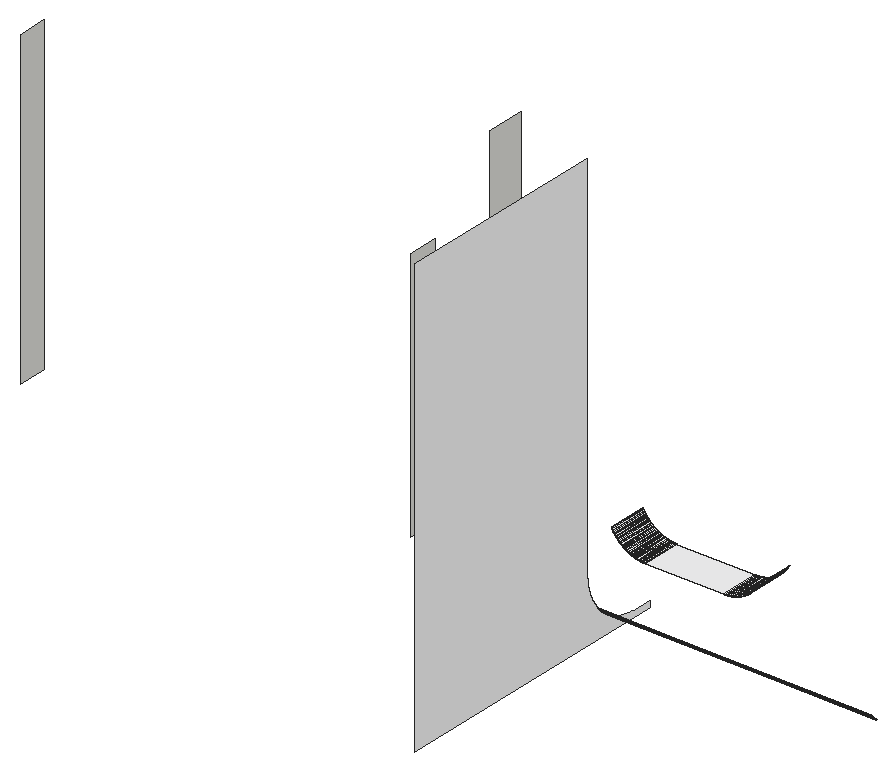
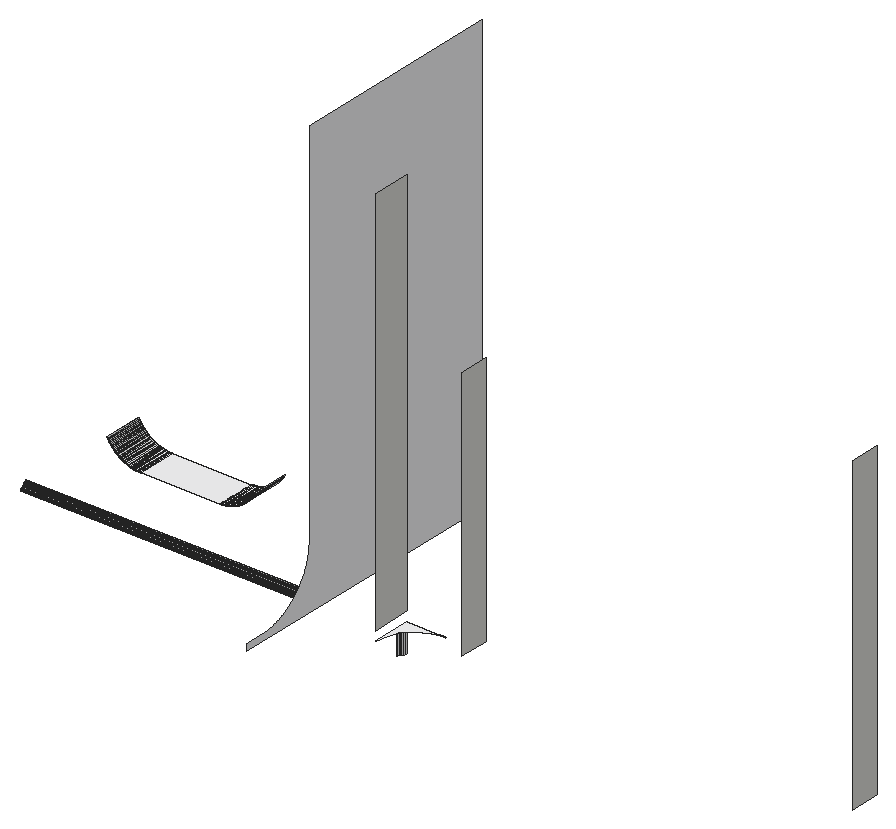
# SketchUp Ruby script. Lengths in inches.
U = 1.inch
M = Sketchup.active_model
def pt(a) = Geom::Point3d.new(a.map { |v| v * U })
def face(e, loops, mat)
  f = e.add_face(loops[0].map { |a| pt(a) })
  loops[1..].each { |l| e.add_face(l.map { |a| pt(a) }).erase! }
  f.material = f.back_material = mat if mat
  f
end
# faces: each face lists its corners as indices into pts; further lists are holes
def faces(e, pts, list, mat = nil) = list.each { |f| face(e, (f[0].is_a?(Array) ? f : [f]).map { |l| l.map { |i| pts[i] } }, mat) }
# xy, xz, yz: faces in a plane at the given z, y or x. An outline is a flat list of corners, or four numbers for a rectangle; further outlines are holes
def ring(l) = l.size == 4 ? [[l[0], l[1]], [l[2], l[1]], [l[2], l[3]], [l[0], l[3]]] : l.each_slice(2).to_a
def flat(e, list, mat, &to3) = list.each { |f| face(e, (f[0].is_a?(Array) ? f : [f]).map { |l| ring(l).map { |u, v| to3.(u, v) } }, mat) }
def xy(e, z, list, mat = nil) = flat(e, list, mat) { |x, y| [x, y, z] }
def xz(e, y, list, mat = nil) = flat(e, list, mat) { |x, z| [x, y, z] }
def yz(e, x, list, mat = nil) = flat(e, list, mat) { |y, z| [x, y, z] }
def lines(e, pts, list) = list.each { |a, b| e.add_line(pt(pts[a]), pt(pts[b])) }
# prism: a flat outline (further loops are holes) pulled along v
def prism(e, loops, v, mat = nil)
  f = face(e, loops, mat); d = Geom::Vector3d.new(v.map { |x| x * U })
  f.pushpull(f.normal.samedirection?(d) ? d.length : -d.length)
end
def box(e, o, s, mat = nil) = prism(e, [[o, [o[0] + s[0], o[1], o[2]], [o[0] + s[0], o[1] + s[1], o[2]], [o[0], o[1] + s[1], o[2]]]], [0, 0, s[2]], mat)
def at(x, y, z, deg = 0) = Geom::Transformation.translation(pt([x, y, z])) * Geom::Transformation.rotation(ORIGIN, Z_AXIS, deg.degrees)
def axes(o, x, y, z) = Geom::Transformation.new([*x, 0, *y, 0, *z, 0, *pt(o).to_a, 1])
def part(name) = M.definitions.add(name)
# library, detail: a bought-in or finely detailed component or shape, given as its bounding box
def library(name, o, s) = part(name).tap { |d| box(d.entities, o, s) }
def detail(e, o, s) = box(e.add_group.entities, o, s)
def put(e, d, t, mat = nil) = e.add_instance(d, t).tap { |i| i.material = mat if mat }
def group(e, t, mat = nil) = e.add_group.tap { |g| g.transformation = t; g.material = mat if mat }.entities
root = M.entities
M.materials.add("[Quartz Light Grey]").color = [251, 251, 252]
xy(root,123,[[186,271,198,271,198,283,198,282.6875,197.99,282.53,197.98,282.37,197.97,282.22,197.95,281.9,197.93,281.75,197.92,281.59,197.9,281.43,197.875,281.28,197.85,281.12,197.83,280.97,197.8,280.8125,197.77,280.66,197.74,280.51,197.7,280.35,197.67,280.2,197.63,280.05,197.59,279.89,197.51,279.59,197.36,279.14,197.3125,278.99,197.26,278.85,197.2,278.7,197.15,278.55,197.09,278.41,197.03,278.26,196.96,278.12,196.9,277.98,196.83,277.83,196.55,277.27,196.47,277.14,196.39,277,196.3125,276.86,196.23,276.73,196.15,276.6,196.0625,276.46,195.98,276.33,195.8,276.07,195.71,275.95,195.62,275.82,195.52,275.69,195.42,275.57,195.33,275.45,195.23,275.33,195.02,275.09,194.92,274.97,194.8125,274.85,194.7,274.74,194.6,274.625,194.49,274.51,194.375,274.4,194.26,274.3,194.15,274.1875,194.03,274.08,193.91,273.98,193.67,273.77,193.55,273.67,193.43,273.58,193.31,273.48,193.18,273.38,193.05,273.29,192.93,273.2,192.67,273.02,192.54,272.9375,192.4,272.85,192.27,272.77,192.14,272.6875,192,272.61,191.86,272.53,191.73,272.45,191.17,272.17,191.02,272.1,190.88,272.04,190.74,271.97,190.59,271.91,190.45,271.85,190.3,271.8,190.15,271.74,190.01,271.6875,189.86,271.64,189.41,271.49,189.11,271.41,188.95,271.37,188.8,271.33,188.65,271.3,188.49,271.26,188.34,271.23,188.1875,271.2,188.03,271.17,187.88,271.15,187.72,271.125,187.57,271.1,187.41,271.08,187.25,271.07,187.1,271.05,186.78,271.03,186.63,271.02,186.47,271.01,186.3125,271]],"[Quartz Light Grey]")
xy(root,144,[[245.84,271,246,283],[246,271,270,283],[270,271,270.16,283]],"[Quartz Light Grey]")
xy(root,144.01,[[245.53,271,245.6875,283],[270.3125,271,270.47,283]],"[Quartz Light Grey]")
yz(root,54,[[271,126,280,222]])
yz(root,174,[[271,126,280,204]])
yz(root,198,[[271,126,283,246]])
yz(root,228,[[205,115,295,115,295,117,288.77,117,288.53,117.01,288.29,117.01,288.06,117.02,287.82,117.04,287.59,117.06,287.35,117.08,287.12,117.1,286.89,117.125,286.65,117.15,286.42,117.1875,286.19,117.22,285.95,117.26,285.72,117.3,285.49,117.35,285.26,117.39,285.03,117.44,284.8,117.5,284.57,117.55,284.34,117.61,284.12,117.68,283.89,117.74,283.66,117.81,283.4375,117.88,283.22,117.96,282.99,118.03,282.77,118.11,282.55,118.2,282.33,118.28,282.11,118.37,281.9,118.46,281.68,118.56,281.46,118.65,281.25,118.75,281.04,118.86,280.83,118.96,280.41,119.18,280.21,119.3,280,119.41,279.6,119.65,279.4,119.78,279.2,119.9,279,120.03,278.81,120.17,278.61,120.3,278.42,120.4375,278.23,120.58,278.04,120.72,277.86,120.86,277.67,121.01,277.49,121.16,277.31,121.3125,277.13,121.47,276.96,121.625,276.78,121.78,276.61,121.94,276.44,122.11,276.27,122.27,276.11,122.44,275.94,122.61,275.78,122.78,275.625,122.96,275.47,123.13,275.3125,123.31,275.16,123.49,275.01,123.67,274.86,123.86,274.72,124.04,274.58,124.23,274.4375,124.42,274.3,124.61,274.17,124.81,274.03,125,273.9,125.2,273.78,125.4,273.65,125.6,273.41,126,273.3,126.21,273.18,126.41,272.96,126.83,272.86,127.04,272.75,127.25,272.65,127.46,272.56,127.68,272.46,127.9,272.37,128.11,272.28,128.33,272.2,128.55,272.11,128.77,272.03,128.99,271.96,129.22,271.88,129.4375,271.81,129.66,271.74,129.89,271.68,130.12,271.61,130.34,271.55,130.57,271.5,130.8,271.44,131.03,271.39,131.26,271.35,131.49,271.3,131.72,271.26,131.95,271.22,132.19,271.1875,132.42,271.15,132.65,271.125,132.89,271.1,133.12,271.08,133.35,271.06,133.59,271.04,133.82,271.02,134.06,271.01,134.29,271.01,134.53,271,134.77,271,249,205,249]],"[Quartz Light Grey]")
p = [[195.02,275.09,117],[194.92,274.97,117],[194.92,274.97,123],[195.02,275.09,123],[195.125,275.21,117],[195.125,275.21,123],
  [195.23,275.33,117],[195.23,275.33,123],[195.33,275.45,117],[195.33,275.45,123],[195.42,275.57,117],[195.42,275.57,123],
  [195.52,275.69,117],[195.52,275.69,123],[195.62,275.82,117],[195.62,275.82,123],[195.71,275.95,117],[195.71,275.95,123],
  [195.8,276.07,117],[195.8,276.07,123],[195.89,276.2,117],[195.89,276.2,123],[195.98,276.33,117],[195.98,276.33,123],
  [196.0625,276.46,117],[196.0625,276.46,123],[196.15,276.6,117],[196.15,276.6,123],[196.23,276.73,117],[196.23,276.73,123],
  [196.3125,276.86,117],[196.3125,276.86,123],[196.39,277,117],[196.39,277,123],[312,276.96,121.625],[312,276.78,121.78],
  [228,276.78,121.78],[228,276.96,121.625],[312,276.61,121.94],[228,276.61,121.94],[312,276.44,122.11],[228,276.44,122.11],
  [312,276.27,122.27],[228,276.27,122.27],[312,276.11,122.44],[228,276.11,122.44],[312,275.94,122.61],[228,275.94,122.61],
  [312,275.78,122.78],[228,275.78,122.78],[312,275.625,122.96],[228,275.625,122.96],[312,275.47,123.13],[228,275.47,123.13],
  [312,275.3125,123.31],[228,275.3125,123.31],[312,275.16,123.49],[228,275.16,123.49],[312,275.01,123.67],[228,275.01,123.67],
  [312,274.86,123.86],[228,274.86,123.86],[245.06,283,144.04],[244.9,283,144.05],[244.9,271,144.05],[245.06,271,144.04],
  [245.22,283,144.03],[245.22,271,144.03],[245.37,283,144.02],[245.37,271,144.02],[245.53,283,144.01],[245.53,271,144.01],
  [245.84,283,144],[245.6875,283,144.01],[245.6875,271,144.01],[245.84,271,144],[270.3125,283,144.01],[270.16,283,144],
  [270.16,271,144],[270.3125,271,144.01],[270.63,283,144.02],[270.47,283,144.01],[270.47,271,144.01],[270.63,271,144.02],
  [270.78,283,144.03],[270.78,271,144.03],[270.94,283,144.04],[270.94,271,144.04],[271.1,283,144.05],[271.1,271,144.05],
  [244.12,283,144.15],[243.97,283,144.17],[243.97,271,144.17],[244.12,271,144.15],[244.28,283,144.125],[244.28,271,144.125],
  [244.43,283,144.1],[244.43,271,144.1],[244.59,283,144.08],[244.59,271,144.08],[244.75,283,144.07],[244.75,271,144.07],
  [271.25,283,144.07],[271.25,271,144.07],[271.41,283,144.08],[271.41,271,144.08],[271.57,283,144.1],[271.57,271,144.1],
  [271.72,283,144.125],[271.72,271,144.125],[271.88,283,144.15],[271.88,271,144.15],[272.03,283,144.17],[272.03,271,144.17],
  [243.66,283,144.23],[243.51,283,144.26],[243.51,271,144.26],[243.66,271,144.23],[243.8125,283,144.2],[243.8125,271,144.2],
  [272.1875,283,144.2],[272.1875,271,144.2],[272.34,283,144.23],[272.34,271,144.23],[272.49,283,144.26],[272.49,271,144.26],
  [243.2,283,144.33],[243.05,283,144.37],[243.05,271,144.37],[243.2,271,144.33],[243.35,283,144.3],[243.35,271,144.3],
  [272.65,283,144.3],[272.65,271,144.3],[272.8,283,144.33],[272.8,271,144.33],[272.95,283,144.37],[272.95,271,144.37],
  [242.89,283,144.41],[242.74,283,144.45],[242.74,271,144.45],[242.89,271,144.41],[273.11,283,144.41],[273.11,271,144.41],
  [273.26,283,144.45],[273.26,271,144.45],[242.44,283,144.54],[242.29,283,144.59],[242.29,271,144.59],[242.44,271,144.54],
  [242.59,283,144.5],[242.59,271,144.5],[273.41,283,144.5],[273.41,271,144.5],[273.56,283,144.54],[273.56,271,144.54],
  [273.71,283,144.59],[273.71,271,144.59],[242.14,283,144.64],[241.99,283,144.69],[241.99,271,144.69],[242.14,271,144.64],
  [273.86,283,144.64],[273.86,271,144.64],[274.01,283,144.69],[274.01,271,144.69],[241.85,283,144.74],[241.7,283,144.8],
  [241.7,271,144.8],[241.85,271,144.74],[274.15,283,144.74],[274.15,271,144.74],[274.3,283,144.8],[274.3,271,144.8],
  [241.55,283,144.86],[241.55,271,144.86],[274.45,283,144.86],[274.45,271,144.86],[241.41,283,144.91],[241.26,283,144.98],
  [241.26,271,144.98],[241.41,271,144.91],[274.59,283,144.91],[274.59,271,144.91],[274.74,283,144.98],[274.74,271,144.98],
  [241.12,283,145.04],[240.98,283,145.1],[240.98,271,145.1],[241.12,271,145.04],[274.88,283,145.04],[274.88,271,145.04],
  [275.02,283,145.1],[275.02,271,145.1],[240.83,283,145.17],[240.83,271,145.17],[275.17,283,145.17],[275.17,271,145.17],
  [240.69,283,145.24],[240.55,283,145.31],[240.55,271,145.31],[240.69,271,145.24],[275.31,283,145.24],[275.31,271,145.24],
  [275.45,283,145.31],[275.45,271,145.31],[240.41,283,145.38],[240.41,271,145.38],[275.59,283,145.38],[275.59,271,145.38],
  [240.27,283,145.46],[240.27,271,145.46],[275.73,283,145.46],[275.73,271,145.46],[240.14,283,145.53],[240,283,145.61],
  [240,271,145.61],[240.14,271,145.53],[275.86,283,145.53],[275.86,271,145.53],[276,283,145.61],[276,271,145.61],
  [239.86,283,145.6875],[239.86,271,145.6875],[276.14,283,145.6875],[276.14,271,145.6875],[239.73,283,145.77],[239.73,271,145.77],
  [276.27,283,145.77],[276.27,271,145.77],[239.6,283,145.85],[239.6,271,145.85],[276.4,283,145.85],[276.4,271,145.85],
  [239.46,283,145.9375],[239.33,283,146.02],[239.33,271,146.02],[239.46,271,145.9375],[276.54,283,145.9375],[276.54,271,145.9375],
  [276.67,283,146.02],[276.67,271,146.02],[239.2,283,146.11],[239.2,271,146.11],[276.8,283,146.11],[276.8,271,146.11],
  [239.07,283,146.2],[239.07,271,146.2],[276.93,283,146.2],[276.93,271,146.2],[238.95,283,146.29],[238.95,271,146.29],
  [277.05,283,146.29],[277.05,271,146.29],[238.82,283,146.39],[238.82,271,146.39],[277.18,283,146.39],[277.18,271,146.39],
  [238.7,283,146.48],[238.7,271,146.48],[277.3,283,146.48],[277.3,271,146.48],[238.57,283,146.58],[238.57,271,146.58],
  [277.43,283,146.58],[277.43,271,146.58],[238.45,283,146.68],[238.45,271,146.68],[277.55,283,146.68],[277.55,271,146.68],
  [238.33,283,146.77],[238.33,271,146.77],[277.67,283,146.77],[277.67,271,146.77],[238.21,283,146.875],[238.21,271,146.875],
  [277.79,283,146.875],[277.79,271,146.875],[238.09,283,146.98],[238.09,271,146.98],[277.91,283,146.98],[277.91,271,146.98],
  [237.97,283,147.08],[237.97,271,147.08],[278.03,283,147.08],[278.03,271,147.08],[237.85,283,147.1875],[237.85,271,147.1875],
  [278.15,283,147.1875],[278.15,271,147.1875],[237.74,283,147.3],[237.74,271,147.3],[278.26,283,147.3],[278.26,271,147.3],
  [237.63,283,147.41],[237.63,271,147.41],[278.37,283,147.41],[278.37,271,147.41],[237.52,283,147.52],[237.52,271,147.52],
  [278.48,283,147.52],[278.48,271,147.52],[237.4,283,147.63],[237.4,271,147.63],[278.6,283,147.63],[278.6,271,147.63],
  [237.3,283,147.74],[237.3,271,147.74],[278.7,283,147.74],[278.7,271,147.74],[237.1875,283,147.86],[237.1875,271,147.86],
  [278.8125,283,147.86],[278.8125,271,147.86],[237.08,283,147.97],[237.08,271,147.97],[278.92,283,147.97],[278.92,271,147.97],
  [236.98,283,148.09],[236.98,271,148.09],[279.02,283,148.09],[279.02,271,148.09],[236.875,283,148.21],[236.875,271,148.21],
  [279.125,283,148.21],[279.125,271,148.21],[236.77,283,148.33],[236.77,271,148.33],[279.23,283,148.33],[279.23,271,148.33],
  [236.67,283,148.45],[236.67,271,148.45],[279.33,283,148.45],[279.33,271,148.45],[236.58,283,148.57],[236.58,271,148.57],
  [279.42,283,148.57],[279.42,271,148.57],[236.48,283,148.7],[236.48,271,148.7],[279.52,283,148.7],[279.52,271,148.7],
  [236.39,283,148.82],[236.39,271,148.82],[279.61,283,148.82],[279.61,271,148.82],[236.29,283,148.95],[236.29,271,148.95],
  [279.71,283,148.95],[279.71,271,148.95],[236.2,283,149.07],[236.2,271,149.07],[279.8,283,149.07],[279.8,271,149.07],
  [236.11,283,149.2],[236.11,271,149.2],[279.89,283,149.2],[279.89,271,149.2],[236.02,283,149.33],[236.02,271,149.33],
  [279.98,283,149.33],[279.98,271,149.33],[235.9375,283,149.47],[235.9375,271,149.47],[280.0625,283,149.47],[280.0625,271,149.47],
  [235.85,283,149.6],[235.85,271,149.6],[280.15,283,149.6],[280.15,271,149.6],[235.77,283,149.73],[235.77,271,149.73],
  [280.23,283,149.73],[280.23,271,149.73],[235.6875,283,149.87],[235.6875,271,149.87],[280.3125,283,149.87],[280.3125,271,149.87],
  [235.61,283,150],[235.61,271,150],[280.39,283,150],[280.39,271,150],[235.53,283,150.14],[235.53,271,150.14],
  [280.47,283,150.14],[280.47,271,150.14],[235.45,283,150.27],[235.45,271,150.27],[280.55,283,150.27],[280.55,271,150.27]]
faces(root,p,[[0,1,2,3],[4,0,3,5],[6,4,5,7],[8,6,7,9],[10,8,9,11],[12,10,11,13],[14,12,13,15],[16,14,15,17],
  [18,16,17,19],[20,18,19,21],[22,20,21,23],[24,22,23,25],[26,24,25,27],[28,26,27,29],[30,28,29,31],[32,30,31,33],
  [34,35,36,37],[35,38,39,36],[38,40,41,39],[40,42,43,41],[42,44,45,43],[44,46,47,45],[46,48,49,47],[48,50,51,49],
  [50,52,53,51],[52,54,55,53],[54,56,57,55],[56,58,59,57],[58,60,61,59],[62,63,64,65],[66,62,65,67],[68,66,67,69],
  [70,68,69,71],[72,73,74,75],[76,77,78,79],[80,81,82,83],[84,80,83,85],[86,84,85,87],[88,86,87,89],[90,91,92,93],
  [94,90,93,95],[96,94,95,97],[98,96,97,99],[100,98,99,101],[63,100,101,64],[102,88,89,103],[104,102,103,105],[106,104,105,107],
  [108,106,107,109],[110,108,109,111],[112,110,111,113],[114,115,116,117],[118,114,117,119],[91,118,119,92],[120,112,113,121],[122,120,121,123],
  [124,122,123,125],[126,127,128,129],[130,126,129,131],[115,130,131,116],[132,124,125,133],[134,132,133,135],[136,134,135,137],[138,139,140,141],
  [127,138,141,128],[142,136,137,143],[144,142,143,145],[146,147,148,149],[150,146,149,151],[139,150,151,140],[152,144,145,153],[154,152,153,155],
  [156,154,155,157],[158,159,160,161],[147,158,161,148],[162,156,157,163],[164,162,163,165],[166,167,168,169],[159,166,169,160],[170,164,165,171],
  [172,170,171,173],[167,174,175,168],[176,172,173,177],[178,179,180,181],[174,178,181,175],[182,176,177,183],[184,182,183,185],[186,187,188,189],
  [179,186,189,180],[190,184,185,191],[192,190,191,193],[187,194,195,188],[196,192,193,197],[198,199,200,201],[194,198,201,195],[202,196,197,203],
  [204,202,203,205],[199,206,207,200],[208,204,205,209],[206,210,211,207],[212,208,209,213],[214,215,216,217],[210,214,217,211],[218,212,213,219],
  [220,218,219,221],[215,222,223,216],[224,220,221,225],[222,226,227,223],[228,224,225,229],[226,230,231,227],[232,228,229,233],[234,235,236,237],
  [230,234,237,231],[238,232,233,239],[240,238,239,241],[235,242,243,236],[244,240,241,245],[242,246,247,243],[248,244,245,249],[246,250,251,247],
  [252,248,249,253],[250,254,255,251],[256,252,253,257],[254,258,259,255],[260,256,257,261],[258,262,263,259],[264,260,261,265],[262,266,267,263],
  [268,264,265,269],[266,270,271,267],[272,268,269,273],[270,274,275,271],[276,272,273,277],[274,278,279,275],[280,276,277,281],[278,282,283,279],
  [284,280,281,285],[282,286,287,283],[288,284,285,289],[286,290,291,287],[292,288,289,293],[290,294,295,291],[296,292,293,297],[294,298,299,295],
  [300,296,297,301],[298,302,303,299],[304,300,301,305],[302,306,307,303],[308,304,305,309],[306,310,311,307],[312,308,309,313],[310,314,315,311],
  [316,312,313,317],[314,318,319,315],[320,316,317,321],[318,322,323,319],[324,320,321,325],[322,326,327,323],[328,324,325,329],[326,330,331,327],
  [332,328,329,333],[330,334,335,331],[336,332,333,337],[334,338,339,335],[340,336,337,341],[338,342,343,339],[344,340,341,345],[342,346,347,343],
  [348,344,345,349],[346,350,351,347],[352,348,349,353],[350,354,355,351],[356,352,353,357],[354,358,359,355],[360,356,357,361],[358,362,363,359],
  [364,360,361,365],[362,366,367,363],[368,364,365,369],[366,370,371,367],[372,368,369,373],[370,374,375,371],[376,372,373,377],[374,378,379,375],
  [380,376,377,381],[378,382,383,379],[384,380,381,385],[382,386,387,383],[388,384,385,389]],"[Quartz Light Grey]")
